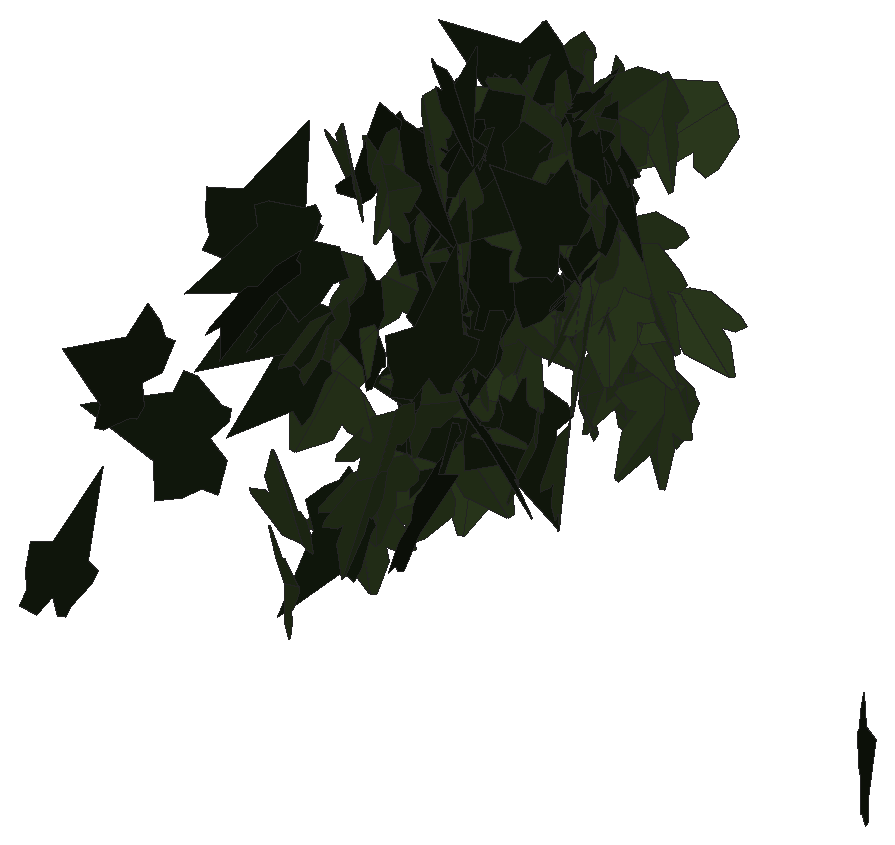
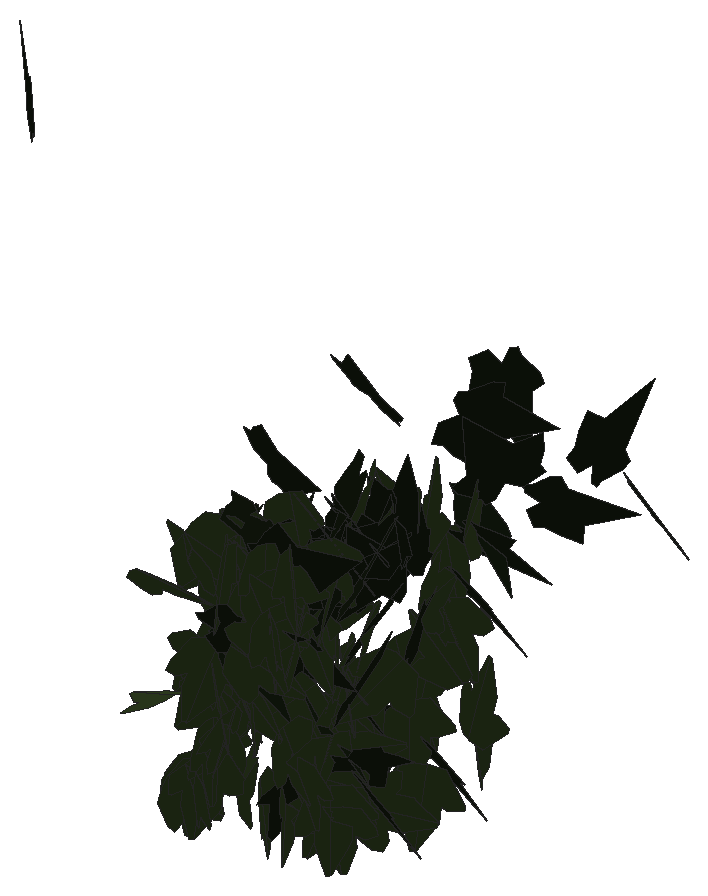
# SketchUp Ruby script. Lengths in inches.
U = 1.inch
M = Sketchup.active_model
def pt(a) = Geom::Point3d.new(a.map { |v| v * U })
def face(e, loops, mat)
  f = e.add_face(loops[0].map { |a| pt(a) })
  loops[1..].each { |l| e.add_face(l.map { |a| pt(a) }).erase! }
  f.material = f.back_material = mat if mat
  f
end
# faces: each face lists its corners as indices into pts; further lists are holes
def faces(e, pts, list, mat = nil) = list.each { |f| face(e, (f[0].is_a?(Array) ? f : [f]).map { |l| l.map { |i| pts[i] } }, mat) }
# xy, xz, yz: faces in a plane at the given z, y or x. An outline is a flat list of corners, or four numbers for a rectangle; further outlines are holes
def ring(l) = l.size == 4 ? [[l[0], l[1]], [l[2], l[1]], [l[2], l[3]], [l[0], l[3]]] : l.each_slice(2).to_a
def flat(e, list, mat, &to3) = list.each { |f| face(e, (f[0].is_a?(Array) ? f : [f]).map { |l| ring(l).map { |u, v| to3.(u, v) } }, mat) }
def xy(e, z, list, mat = nil) = flat(e, list, mat) { |x, y| [x, y, z] }
def xz(e, y, list, mat = nil) = flat(e, list, mat) { |x, z| [x, y, z] }
def yz(e, x, list, mat = nil) = flat(e, list, mat) { |y, z| [x, y, z] }
def lines(e, pts, list) = list.each { |a, b| e.add_line(pt(pts[a]), pt(pts[b])) }
# prism: a flat outline (further loops are holes) pulled along v
def prism(e, loops, v, mat = nil)
  f = face(e, loops, mat); d = Geom::Vector3d.new(v.map { |x| x * U })
  f.pushpull(f.normal.samedirection?(d) ? d.length : -d.length)
end
def box(e, o, s, mat = nil) = prism(e, [[o, [o[0] + s[0], o[1], o[2]], [o[0] + s[0], o[1] + s[1], o[2]], [o[0], o[1] + s[1], o[2]]]], [0, 0, s[2]], mat)
def at(x, y, z, deg = 0) = Geom::Transformation.translation(pt([x, y, z])) * Geom::Transformation.rotation(ORIGIN, Z_AXIS, deg.degrees)
def axes(o, x, y, z) = Geom::Transformation.new([*x, 0, *y, 0, *z, 0, *pt(o).to_a, 1])
def part(name) = M.definitions.add(name)
# library, detail: a bought-in or finely detailed component or shape, given as its bounding box
def library(name, o, s) = part(name).tap { |d| box(d.entities, o, s) }
def detail(e, o, s) = box(e.add_group.entities, o, s)
def put(e, d, t, mat = nil) = e.add_instance(d, t).tap { |i| i.material = mat if mat }
def group(e, t, mat = nil) = e.add_group.tap { |g| g.transformation = t; g.material = mat if mat }.entities
root = M.entities
M.materials.add("efeu1").color = [18, 25, 13]
M.materials.add("efeu2").color = [43, 57, 29]
c1 = part("ivyleaf_10")
p = [[0,0.5,-0.03],[-0.0625,2.02,-0.43],[-0.19,2.01,-0.46],[-0.54,1.05,-0.29],[-0.52,0.625,-0.18],[-0.83,0.76,-0.28],
  [-1.16,0.64,-0.33],[-1.15,0.33,-0.24],[-0.77,-0.39,0.02],[-0.3,-0.51,0.16],[0.04,-0.48,0.23],[-0.02,2.01,-0.4375],
  [-0.06,2.01,-0.43],[0.04,-0.49,0.23],[0.67,-0.49,0.14],[1.38,0.36,-0.2],[1.375,0.51,-0.24],[0.81,0.65,-0.19],
  [0.62,0.59,-0.15],[0.6,1.09,-0.28],[0.5,1.23,-0.31]]
faces(c1.entities,p,[[0,1,2,3,4,5,6,7,8,9,10],[11,12,0,13,14,15,16,17,18,19,20]],"efeu2")
c2 = part("ivyleaf_9")
p = [[1.54,2.16,1.25],[1.36,2.04,1.19],[-0.21,0.99,0.68],[-0.71,1.11,0.82],[-0.85,0.86,0.67],[-0.8,0.17,0.21],
  [-0.9,-0.01,0.1],[-0.67,-0.16,-0.02],[-0.08,-0.08,-0.05],[-0.03,-0.6,-0.4],[0.65,-0.88,-0.66],[0.83,-0.6,-0.49],
  [1.29,-0.42,-0.43],[1.8125,-0.07,-0.26],[1.21,0.44,0.15]]
faces(c2.entities,p,[[0,1,2,3,4,5,6,7,8,9,10,11,12,13,14]],"efeu1")
p = [[2418.138,81.9375,201.614],[2418.14,81.9375,201.614],[2416.236,75.319,201.631],[2416.239,75.323,201.633]]
lines(root,p,[[0,1],[2,3]])
put(root,c1,axes([53.28,224.05,204.59],[-0.23374,-0.23378,-0.37512],[0.25707,0.27328,-0.3305],[0.35955,-0.34737,-0.00756]))
put(root,c2,axes([53.61,224.3,202.78],[-0.47909,0.10832,-0.09347],[0.08974,-0.02688,-0.49115],[-0.11142,-0.48739,0.00631]))
put(root,c1,axes([53.48,222.9375,206.35],[-0.4085,0.26091,0.12269],[0.10303,-0.06662,0.48471],[0.26928,0.42129,0.00067]))
put(root,c2,axes([53.64,224.5,204.12],[-0.05286,-0.45379,0.20317],[0.04876,0.1986,0.45627],[-0.4948,0.06805,0.02326]))
put(root,c1,axes([53.62,221.7,202.63],[-0.47006,0.16487,-0.04318],[-0.04138,0.01247,0.49813],[0.16533,0.47187,0.00192]))
put(root,c2,axes([53.45,223.6,206.18],[0.25603,0.25764,0.34361],[-0.23181,-0.25385,0.36307],[0.36154,-0.34523,-0.01054]))
put(root,c2,axes([53.81,221.64,205.58],[-0.4854,-0.05753,0.10523],[-0.10052,-0.04412,-0.4878],[0.06541,-0.49472,0.03127]))
put(root,c2,axes([53.48,221.24,206.4],[-0.22906,-0.15237,0.41751],[0.37864,0.17905,0.27308],[-0.23273,0.44127,0.03336]))
put(root,c2,axes([53.63,218.98,205.67],[0.03394,0.03629,0.49752],[-0.31738,-0.38316,0.0496],[0.38486,-0.31918,-0.00297]))
put(root,c1,axes([53.79,223.88,202.12],[-0.07725,-0.12335,0.47835],[-0.22753,-0.42087,-0.14527],[0.43848,-0.24012,0.0089]))
put(root,c1,axes([53.63,222.89,202.17],[-0.47639,-0.15179,-0.00356],[0.00396,-0.00069,-0.49998],[0.15178,-0.4764,0.00186]))
put(root,c1,axes([53.4,222.08,205.98],[-0.02157,0.03447,0.49834],[0.33654,-0.36762,0.04],[0.36916,0.33715,-0.00734]))
put(root,c1,axes([53.69,223.96,205.26],[-0.26767,0.36628,0.21022],[-0.1167,0.17505,-0.45359],[-0.40588,-0.29189,-0.00822]))
put(root,c1,axes([53.35,222.61,203.97],[0.39116,-0.05211,-0.30705],[0.30426,-0.04132,0.39461],[-0.06651,-0.49556,-0.00062]))
put(root,c2,axes([53.87,221.71,204.84],[-0.48279,0.12763,-0.025],[0.0236,-0.00853,-0.49937],[-0.1279,-0.48336,0.00221]))
put(root,c2,axes([53.46,224.1,205.46],[0.26682,-0.38122,-0.18298],[-0.10109,0.15258,-0.46529],[0.4106,0.28529,0.00435]))
put(root,c2,axes([53.62,224.55,203.29],[-0.31701,-0.38257,-0.05611],[0.08209,0.00431,-0.4932],[0.37785,-0.3219,0.06008]))
put(root,c1,axes([53.8,225.72,206.86],[-0.18704,0.45163,0.10509],[-0.2191,0.0138,-0.44923],[-0.40867,-0.2141,0.19274]))
put(root,c2,axes([53.94,221.26,205.83],[-0.22957,0.43587,0.08553],[-0.06038,0.06476,-0.4921],[-0.44006,-0.23627,0.0229]))
put(root,c2,axes([53.6,223.18,204.45],[-0.05861,-0.04775,0.49425],[-0.08765,-0.48887,-0.05762],[0.48876,-0.0934,0.04894]))
put(root,c2,axes([53.84,222.48,202.47],[-0.48202,0.06943,-0.11329],[0.11037,-0.02816,-0.48685],[-0.07399,-0.49435,0.01182]))
put(root,c1,axes([53.79,224.68,206.27],[-0.26166,0.31803,0.28353],[-0.17814,0.22059,-0.41183],[-0.38704,-0.31653,-0.00213]))
put(root,c2,axes([53.74,224.53,205.74],[0.18724,-0.46327,0.0181],[0.00999,0.02354,0.49935],[-0.46351,-0.18663,0.01807]))
put(root,c1,axes([53.97,224.45,203.2],[0.06499,0.09954,0.48566],[-0.32401,-0.3622,0.11759],[0.37523,-0.33,0.01742]))
put(root,c1,axes([53.76,226.08,206.05],[-0.10332,-0.48388,0.07198],[0.01088,-0.07582,-0.4941],[0.48909,-0.10054,0.0262]))
put(root,c1,axes([53.77,224.79,202.59],[-0.25234,-0.43045,-0.03219],[0.00979,0.03156,-0.49891],[0.43154,-0.25242,-0.0075]))
put(root,c2,axes([53.7,223.88,205.76],[-0.16584,-0.23251,0.41041],[0.30625,0.27781,0.28113],[-0.35876,0.34462,0.05027]))
put(root,c2,axes([54.09,225.51,206.54],[-0.06941,0.01806,0.49483],[-0.4596,0.18359,-0.07117],[-0.18426,-0.46472,-0.00888]))
put(root,c1,axes([53.58,222.8,205.08],[0.02326,-0.0361,0.49815],[0.2512,-0.43019,-0.04291],[0.43169,0.25226,-0.00187]))
put(root,c1,axes([53.83,225.45,205.35],[-0.12511,0.45102,-0.17586],[-0.0539,0.16754,0.468],[0.48108,0.13606,0.00669]))
put(root,c2,axes([53.8,217.27,203.82],[-0.36243,0.33161,0.09319],[0.06684,-0.06499,0.49123],[0.3379,0.36853,0.00278]))
put(root,c1,axes([53.76,223.4,206.66],[0.00014,0.42659,-0.26081],[-0.04813,-0.25959,-0.42462],[-0.49768,0.02523,0.04099]))
put(root,c1,axes([53.92,221.9375,204.35],[0.43854,0.13261,-0.20024],[-0.22884,0.10421,-0.43217],[-0.07288,0.4707,0.15209]))
put(root,c1,axes([53.75,224.73,202.35],[0.44618,0.22492,-0.01834],[-0.01561,-0.00978,-0.49966],[-0.22513,0.44645,-0.0017]))
put(root,c2,axes([54.2,219.41,204.96],[-0.24741,-0.20426,-0.38349],[-0.27518,-0.26785,0.32021],[-0.33625,0.36951,0.02012]))
put(root,c2,axes([53.73,223.75,206.25],[0.33823,0.35681,0.09107],[0.05963,0.06896,-0.49162],[-0.36338,0.34342,0.00409]))
put(root,c1,axes([53.58,221.59,201.91],[-0.22194,0.12447,0.4304],[0.38348,-0.19561,0.25432],[0.2317,0.44299,-0.00864]))
put(root,c1,axes([53.9,225.79,206.52],[-0.29571,-0.40198,0.03107],[0.0206,-0.05355,-0.4967],[0.40265,-0.29248,0.04823]))
put(root,c1,axes([53.8,226.04,206.01],[0.32534,-0.37868,0.02749],[0.09127,0.04286,-0.48973],[0.36854,0.32367,0.09701]))
put(root,c1,axes([53.8,224.85,203.53],[0.10436,0.48338,0.07383],[0.0158,0.07212,-0.49452],[-0.48873,0.10555,-0.00022]))
put(root,c1,axes([53.82,226.08,205.9],[-0.21811,-0.43033,0.13134],[0.06394,0.11483,0.48242],[-0.44535,0.22723,0.00494]))
put(root,c1,axes([53.99,224.85,206.58],[0.40906,0.19044,-0.21542],[-0.19342,-0.09492,-0.4512],[-0.21275,0.45246,-0.00399]))
put(root,c1,axes([54.02,224.5,203.79],[-0.19514,0.36351,0.28245],[-0.16364,0.23197,-0.4116],[-0.43028,-0.25308,0.02844]))
put(root,c1,axes([54.01,224.15,204.5],[0.21719,-0.42305,-0.15445],[-0.06098,0.14226,-0.47544],[0.44622,0.22536,0.0102]))
put(root,c1,axes([53.95,224.2,204.7],[-0.24271,0.43215,0.06589],[-0.03468,0.05609,-0.49563],[-0.43576,-0.24516,0.00274]))
put(root,c1,axes([54.22,224.84,205.35],[-0.39501,-0.04351,0.30343],[-0.29888,-0.05526,-0.39701],[0.06808,-0.49503,0.01765]))
put(root,c1,axes([54.06,225.89,206.19],[-0.11148,-0.35076,0.33843],[-0.04381,-0.33856,-0.36532],[0.48544,-0.11111,0.04475]))
put(root,c1,axes([53.8,224.71,205.16],[0.10773,-0.29284,-0.39069],[0.13227,-0.36763,0.31202],[-0.47,-0.17058,-0.00174]))
put(root,c1,axes([54.04,222.66,202.96],[-0.20056,-0.45575,-0.04549],[0.00821,0.04608,-0.4978],[0.45794,-0.20043,-0.011]))
put(root,c1,axes([53.98,225.23,203.3],[0.47455,-0.15312,-0.03679],[-0.03346,0.01612,-0.49862],[0.15388,0.4757,0.00506]))
put(root,c2,axes([54.06,223.75,206.35],[-0.40737,0.28322,0.06195],[0.04763,-0.04001,0.49611],[0.28598,0.41011,0.00562]))
put(root,c1,axes([54,224.35,203.98],[0.04492,-0.36389,0.33995],[0.05597,-0.33547,-0.3665],[0.49482,0.07098,0.01059]))
put(root,c1,axes([54.0625,225.33,203.72],[-0.00044,-0.48437,0.12404],[0.00328,-0.12404,-0.48436],[0.49999,0.00038,0.00328]))
put(root,c1,axes([54.07,221.71,205.31],[0.00059,-0.4999,-0.00987],[0.00881,0.00988,-0.49982],[0.49992,0.00041,0.00882]))
put(root,c2,axes([53.6875,223.5,206.69],[-0.01887,-0.02168,-0.49917],[0.48587,0.1157,-0.02339],[0.11652,-0.48595,0.0167]))
put(root,c1,axes([54,224.38,202.51],[-0.35788,-0.29109,-0.19285],[0.15332,0.11711,-0.46128],[0.31371,-0.3893,0.00543]))
put(root,c1,axes([54.42,225.93,205.25],[-0.16154,-0.04782,0.47076],[-0.42513,-0.20376,-0.16658],[0.20777,-0.45409,0.02517]))
put(root,c1,axes([54.09,223.5,203.59],[-0.0181,-0.22121,-0.44804],[0.04357,0.44593,-0.22192],[0.49777,-0.04708,0.00313]))
put(root,c2,axes([54.31,224.43,203.97],[-0.38545,0.31485,-0.04795],[0.0377,-0.02964,-0.49769],[-0.31624,-0.38729,-0.0009]))
put(root,c2,axes([54.23,224.27,204.4],[-0.48497,0.03456,-0.11666],[0.11473,-0.02965,-0.48575],[-0.04049,-0.49792,0.02083]))
put(root,c1,axes([53.81,223.1,206.3],[-0.28107,0.04516,0.41105],[0.40309,-0.08099,0.28453],[0.09228,0.49133,0.00912]))
put(root,c1,axes([54.1,225.83,206.86],[-0.09176,-0.48397,-0.08577],[0.05515,0.07656,-0.49102],[0.4884,-0.09957,0.03933]))
put(root,c1,axes([54.16,224.64,205.36],[-0.0183,-0.01614,0.4994],[-0.00882,-0.49965,-0.01647],[0.49959,-0.00941,0.018]))
put(root,c2,axes([53.84,224.75,206.1],[0.46189,-0.19107,-0.01231],[-0.01075,0.0062,-0.49985],[0.19117,0.46201,0.00162]))
put(root,c1,axes([54.0625,223.6,207.11],[-0.1851,0.45365,-0.09972],[0.03814,-0.09214,-0.48995],[-0.46291,-0.18898,-0.00049]))
put(root,c2,axes([54.5,224.23,206.6875],[-0.34906,0.28633,0.21487],[-0.16595,0.13649,-0.45148],[-0.3172,-0.3865,-0.00025]))
put(root,c2,axes([54.08,223.83,207.33],[0.38775,-0.12928,-0.28799],[-0.25693,0.13577,-0.40688],[0.1834,0.46352,0.03885]))
put(root,c1,axes([54.23,225.25,206.39],[-0.02413,-0.46096,0.19218],[-0.01225,-0.1918,-0.46159],[0.49927,-0.02699,-0.00204]))
put(root,c2,axes([54.2,224.35,206.54],[-0.13,0.20227,-0.43839],[0.23399,-0.37073,-0.24044],[-0.42231,-0.26768,0.00173]))
put(root,c2,axes([54.28,224.73,204.64],[-0.00217,0.06605,0.49561],[-0.25476,-0.42661,0.05574],[0.43023,-0.25228,0.0355]))
put(root,c2,axes([54.65,224.79,205],[-0.15127,0.01284,-0.4764],[-0.42479,-0.2302,0.12868],[-0.21602,0.44367,0.08055]))
put(root,c1,axes([54.29,222.16,203.06],[0.05456,-0.48122,0.12429],[0.04081,-0.12028,-0.4836],[0.49534,0.06292,0.02615]))
put(root,c1,axes([54.35,222.47,203.81],[-0.04431,-0.49491,0.05567],[0.00176,-0.05605,-0.49685],[0.49803,-0.04384,0.00671]))
put(root,c2,axes([54.52,220.84,206.91],[-0.05705,-0.11709,-0.48274],[-0.05597,-0.4813,0.12336],[-0.49357,0.06811,0.04181]))
put(root,c2,axes([54.17,224.89,202.93],[0.05162,-0.41923,-0.26754],[-0.02114,0.26689,-0.42229],[0.49688,0.05491,0.00983]))
put(root,c1,axes([54.42,224.92,202.57],[0.09295,-0.38185,-0.30912],[-0.06368,0.30258,-0.39292],[0.48714,0.11241,0.00762]))
put(root,c1,axes([54.13,223.93,206.2],[0.41917,-0.13227,0.23832],[0.23072,-0.0606,-0.43943],[0.14513,0.47836,0.01023]))
put(root,c2,axes([54.78,226.04,205.62],[-0.29794,-0.20639,-0.34443],[-0.28326,-0.19596,0.36244],[-0.2846,0.4111,-0.00015]))
put(root,c1,axes([54.66,224.61,206.97],[-0.44343,0.01014,0.2308],[-0.231,-0.02652,-0.44265],[0.00327,-0.49919,0.02821]))
put(root,c1,axes([54.25,224.86,204.26],[-0.35123,-0.04463,-0.35305],[0.3535,0.01326,-0.35336],[0.04091,-0.49783,0.02224]))
put(root,c1,axes([54.53,225.42,205.98],[-0.29428,-0.40178,-0.04442],[0.03072,0.03256,-0.49799],[0.40306,-0.29583,0.00552]))
put(root,c1,axes([54.78,225.47,202.83],[-0.22779,0.29264,-0.33537],[-0.19405,0.27375,0.37068],[0.40057,0.29903,-0.01115]))
put(root,c2,axes([54.74,222.43,202.79],[-0.1244,0.17301,-0.45232],[-0.32961,0.31189,0.20995],[0.35479,0.35042,0.03646]))
put(root,c1,axes([54.61,225.17,206.62],[0.13504,-0.29272,-0.38221],[0.01914,0.39991,-0.29951],[0.48104,0.06626,0.11921]))
put(root,c1,axes([54.97,225.35,204.28],[-0.17479,0.04171,0.46659],[-0.46832,-0.00346,-0.17513],[-0.01138,-0.49825,0.04028]))
put(root,c2,axes([54.83,219.57,207.01],[-0.1274,0.45928,-0.15109],[0.04058,-0.14554,-0.47662],[-0.48179,-0.13371,-0.0002]))
put(root,c1,axes([55.04,224.4,205.65],[-0.09623,-0.02062,-0.49022],[-0.46892,-0.14317,0.09807],[-0.14441,0.47862,0.00821]))
put(root,c2,axes([54.93,224.89,206.79],[-0.01149,0.44752,0.22269],[-0.13415,0.21182,-0.43259],[-0.48153,-0.06969,0.1152]))
put(root,c1,axes([54.92,225.67,206.37],[-0.35956,-0.22294,0.26649],[-0.18748,-0.19838,-0.41892],[0.29252,-0.40118,0.05907]))
put(root,c2,axes([54.93,224.41,206.38],[-0.4374,-0.19354,0.14567],[-0.12344,-0.08062,-0.47777],[0.20843,-0.45392,0.02275]))
put(root,c1,axes([54.84,225.16,204.36],[0.11896,-0.41254,-0.25624],[-0.07501,0.24504,-0.42934],[0.47981,0.14059,-0.00359]))
put(root,c1,axes([54.74,225.91,206.66],[0.14823,-0.4437,-0.17652],[0.07309,0.20373,-0.45072],[0.4719,0.10781,0.12526]))
put(root,c1,axes([54.73,225.09,202.55],[0.20264,-0.45416,0.05172],[0.10273,-0.00987,-0.48923],[0.4454,0.2089,0.08931]))
put(root,c2,axes([55.14,225.17,204.99],[-0.29366,0.39542,-0.08606],[-0.01465,-0.11665,-0.48598],[-0.40441,-0.28291,0.0801]))
put(root,c2,axes([55.22,225.1,206.4],[-0.42528,0.23367,0.12055],[-0.10058,0.06722,-0.48514],[-0.24293,-0.4369,-0.01017]))
put(root,c1,axes([54.98,225.24,206.7],[-0.01864,-0.49965,0.00196],[-0.00027,-0.00195,-0.5],[0.49965,-0.01864,-0.00019]))
put(root,c1,axes([55.06,225.72,204.57],[0.20167,-0.43076,-0.15419],[-0.06693,0.13892,-0.47563],[0.4526,0.21248,-0.00163]))
put(root,c1,axes([54.96,225.65,203.89],[-0.11055,0.485,0.05058],[-0.00923,0.04977,-0.49743],[-0.48754,-0.11091,-0.00205]))
put(root,c1,axes([55.07,225.69,203.64],[0.0954,0.43617,-0.22506],[-0.14936,-0.1926,-0.43657],[-0.46754,0.15053,0.09354]))
put(root,c1,axes([55.26,225.9,206.84],[0.18868,0.27938,-0.36925],[-0.3698,-0.14903,-0.30173],[-0.27866,0.38695,0.15039]))
put(root,c1,axes([54.82,225.07,204.68],[-0.03155,-0.20687,-0.4541],[0.23512,-0.4075,0.1693],[-0.44014,-0.20285,0.12299]))
put(root,c1,axes([55.22,224.9,206.39],[-0.14179,0.19303,0.4389],[-0.24095,0.36702,-0.23925],[-0.41454,-0.27935,-0.01106]))
put(root,c1,axes([54.91,225.47,206.15],[-0.40509,0.02573,0.29195],[0.28607,-0.07358,0.40342],[0.06373,0.49389,0.04489]))
put(root,c2,axes([55.05,224.5,205.54],[0.3177,-0.38399,0.04027],[-0.01368,0.04093,0.49813],[-0.38585,-0.31762,0.0155]))
put(root,c1,axes([55.1,225.5,205.9],[-0.02717,-0.25822,0.4273],[0.08242,-0.42438,-0.25122],[0.49241,0.05678,0.06563]))
put(root,c1,axes([55.07,225.84,204.99],[-0.35728,-0.30397,-0.17307],[0.14512,0.09628,-0.46869],[0.31826,-0.38514,0.01943]))
put(root,c1,axes([55,224.36,206.11],[-0.09081,-0.19238,-0.45249],[0.22303,0.39396,-0.21225],[0.43819,-0.24039,0.01426]))
put(root,c1,axes([55.13,225.71,203.63],[-0.04406,-0.49282,-0.07204],[0.0528,0.06729,-0.49263],[0.49525,-0.05102,0.04612]))
put(root,c1,axes([54.9375,225.22,204.1],[0.26301,-0.2339,0.35513],[0.25072,-0.25197,-0.35164],[0.34346,0.36305,-0.01526]))
put(root,c2,axes([55.27,225.24,205.79],[-0.42579,0.1372,-0.22334],[0.20843,-0.08111,-0.44719],[-0.15894,-0.47392,0.01188]))
put(root,c1,axes([55.17,225.33,205.09],[0.493,0.02858,-0.0783],[-0.07895,0.00951,-0.49364],[-0.02673,0.49909,0.01389]))
put(root,c1,axes([55.21,225.86,203.13],[-0.37971,-0.31973,-0.05992],[0.04514,0.03942,-0.4964],[0.32215,-0.38239,-0.00107]))
put(root,c1,axes([55.16,225.33,204.48],[0.35542,0.35121,0.01809],[0.01294,0.01264,-0.49967],[-0.35144,0.35566,-0.00011]))
put(root,c1,axes([55.3,226.0625,202.93],[-0.45731,0.17183,-0.10649],[0.03725,-0.18724,-0.46212],[-0.19869,-0.4306,0.15846]))
put(root,c1,axes([55.25,225.32,205.25],[-0.21907,0.30417,0.3309],[0.19699,-0.26589,0.37483],[0.40399,0.29459,-0.00334]))
put(root,c1,axes([55.62,226.56,206.38],[-0.40111,0.18698,0.2327],[-0.27246,-0.38858,-0.15739],[0.12199,-0.25306,0.41362]))
put(root,c1,axes([55.43,226.1,202.9],[-0.11529,-0.32457,0.36244],[-0.00039,-0.37241,-0.33363],[0.48653,-0.0772,0.08562]))
put(root,c2,axes([55.17,225.17,206.54],[0.24717,-0.43144,0.0526],[0.02817,-0.04448,-0.49722],[0.43372,0.24876,0.00232]))
put(root,c1,axes([55.18,225.63,204.22],[0.34383,0.07196,0.35581],[0.33992,0.10819,-0.35036],[-0.12741,0.48282,0.02548]))
put(root,c1,axes([55.25,226.07,206.68],[0.39766,-0.08113,0.29203],[0.28566,-0.06069,-0.40585],[0.1013,0.48963,-0.00192]))
put(root,c1,axes([55.41,225.69,204.79],[-0.39092,0.11816,-0.28848],[0.2373,-0.18728,-0.39827],[-0.20217,-0.44829,0.09034]))
put(root,c2,axes([56.21,223.12,206.53],[-0.13336,0.16126,0.4541],[-0.31906,0.32355,-0.2086],[-0.36113,-0.34541,0.01661]))
put(root,c2,axes([55.63,222.53,204.21],[0.22978,-0.32968,0.29751],[0.17428,-0.24115,-0.40183],[0.40844,0.28837,0.00409]))
put(root,c1,axes([55.72,226.06,204.2],[-0.20137,-0.45754,0.01029],[0.45103,-0.2003,-0.08033],[0.07763,-0.02307,0.4934]))
put(root,c2,axes([56.68,220.3,206.27],[-0.44293,0.22904,0.03681],[0.03272,-0.01687,0.49864],[0.22967,0.44413,-0.00004]))
put(root,c2,axes([65.7,216.66,205.95],[-0.02274,0.12913,0.4825],[0.08649,-0.47469,0.13112],[0.49194,0.08942,-0.00075]))
